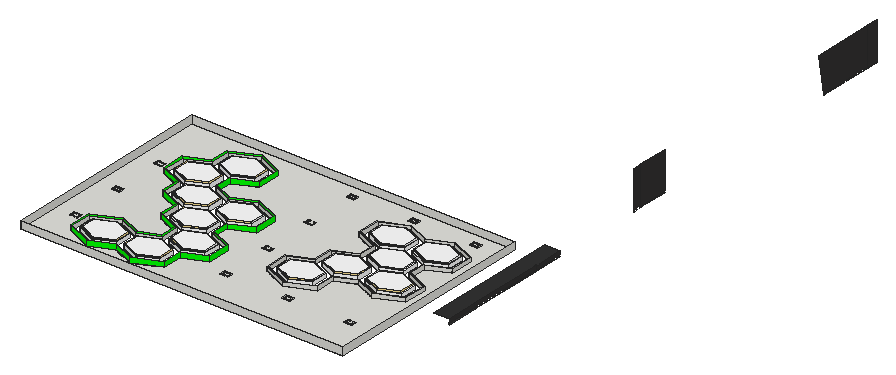
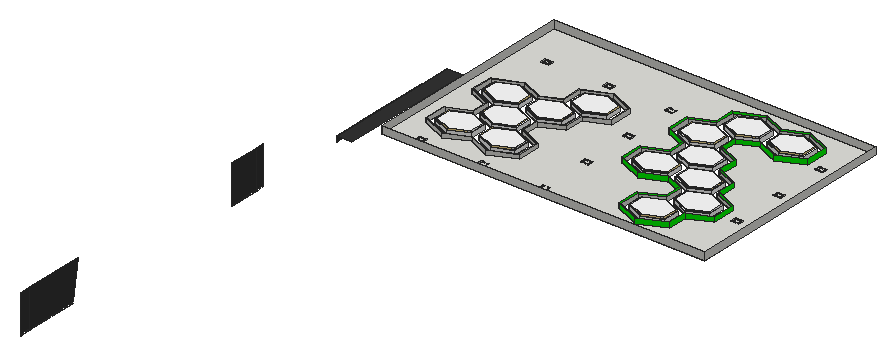
# SketchUp Ruby script. Lengths in inches.
U = 1.inch
M = Sketchup.active_model
def pt(a) = Geom::Point3d.new(a.map { |v| v * U })
def face(e, loops, mat)
  f = e.add_face(loops[0].map { |a| pt(a) })
  loops[1..].each { |l| e.add_face(l.map { |a| pt(a) }).erase! }
  f.material = f.back_material = mat if mat
  f
end
# faces: each face lists its corners as indices into pts; further lists are holes
def faces(e, pts, list, mat = nil) = list.each { |f| face(e, (f[0].is_a?(Array) ? f : [f]).map { |l| l.map { |i| pts[i] } }, mat) }
# xy, xz, yz: faces in a plane at the given z, y or x. An outline is a flat list of corners, or four numbers for a rectangle; further outlines are holes
def ring(l) = l.size == 4 ? [[l[0], l[1]], [l[2], l[1]], [l[2], l[3]], [l[0], l[3]]] : l.each_slice(2).to_a
def flat(e, list, mat, &to3) = list.each { |f| face(e, (f[0].is_a?(Array) ? f : [f]).map { |l| ring(l).map { |u, v| to3.(u, v) } }, mat) }
def xy(e, z, list, mat = nil) = flat(e, list, mat) { |x, y| [x, y, z] }
def xz(e, y, list, mat = nil) = flat(e, list, mat) { |x, z| [x, y, z] }
def yz(e, x, list, mat = nil) = flat(e, list, mat) { |y, z| [x, y, z] }
def lines(e, pts, list) = list.each { |a, b| e.add_line(pt(pts[a]), pt(pts[b])) }
# prism: a flat outline (further loops are holes) pulled along v
def prism(e, loops, v, mat = nil)
  f = face(e, loops, mat); d = Geom::Vector3d.new(v.map { |x| x * U })
  f.pushpull(f.normal.samedirection?(d) ? d.length : -d.length)
end
def box(e, o, s, mat = nil) = prism(e, [[o, [o[0] + s[0], o[1], o[2]], [o[0] + s[0], o[1] + s[1], o[2]], [o[0], o[1] + s[1], o[2]]]], [0, 0, s[2]], mat)
def at(x, y, z, deg = 0) = Geom::Transformation.translation(pt([x, y, z])) * Geom::Transformation.rotation(ORIGIN, Z_AXIS, deg.degrees)
def axes(o, x, y, z) = Geom::Transformation.new([*x, 0, *y, 0, *z, 0, *pt(o).to_a, 1])
def part(name) = M.definitions.add(name)
# library, detail: a bought-in or finely detailed component or shape, given as its bounding box
def library(name, o, s) = part(name).tap { |d| box(d.entities, o, s) }
def detail(e, o, s) = box(e.add_group.entities, o, s)
def put(e, d, t, mat = nil) = e.add_instance(d, t).tap { |i| i.material = mat if mat }
def group(e, t, mat = nil) = e.add_group.tap { |g| g.transformation = t; g.material = mat if mat }.entities
root = M.entities
M.materials.add("False Ceiling Light").color = [250, 224, 145]
M.materials.add("[0128_White]1").color = [255, 255, 255]
M.materials.add("[Color G05]").color = [0, 255, 0]
M.materials.add("[Granite Dark Gray]").color = [51, 50, 50]
c1 = part("Group1089\#2")
p = [[0,0,0],[0,0,-1.54],[-0.31,0,-1.54],[2,-3,0],[-2,-3,0],[2,3,0],
  [2,0,0],[-2,3,0],[0.31,0,-1.54],[-2,0,0],[0,0,-2.5]]
lines(c1.entities,p,[[0,1],[1,2],[3,4],[5,6],[7,5],[1,8],[9,0],[0,6],[8,10],[4,9],[6,3],[2,10],
  [9,7]])
c2 = part("Rectangle Light")
put(c2.entities,c1,at(0,0,0))
c3 = part("Group823\#1")
xy(c3.entities,0,[[-3,-3,3,3]])
put(c3.entities,c2,axes([0,0,-0.01],[1.3627,0,0],[0,1.90637,0],[0,0,1.35135]))
c4 = part("HUY")
xy(c4.entities,0,[[[-1,-1,7,7],[0,0,6,6]]])
xy(c4.entities,0.1,[[0,0,6,6]])
xy(c4.entities,0.6,[[[-1,-1,7,7],[0,0,6,6]]])
xz(c4.entities,-1,[[-1,0,7,0.6]])
xz(c4.entities,0,[[0,0,6,0.1],[0,0.1,6,0.6]])
xz(c4.entities,6,[[0,0,6,0.1],[0,0.1,6,0.6]])
xz(c4.entities,7,[[-1,0,7,0.6]])
yz(c4.entities,-1,[[-1,0,7,0.6]])
yz(c4.entities,0,[[0,0,6,0.1],[0,0.1,6,0.6]])
yz(c4.entities,6,[[0,0,6,0.1],[0,0.1,6,0.6]])
yz(c4.entities,7,[[-1,0,7,0.6]])
put(c4.entities,c3,axes([3,3,0.6],[1,0,0],[0,1,0],[0,0,-1]))
c5 = part("Group849\#3")
xy(c5.entities,0,[[-15.5,-0.5,15.5,0.5]])
c6 = part("Group849\#6")
xy(c6.entities,0,[[-15.5,-0.5,15.5,0.5]])
c7 = part("Group849\#4")
xy(c7.entities,0,[[-15.5,-0.5,15.5,0.5]])
c8 = part("Group849\#5")
xy(c8.entities,0,[[-15.5,-0.5,15.5,0.5]])
c9 = part("HEXAGON")
xy(c9.entities,0,[[15.59,1.15,1,9.58,1,26.42,15.59,34.85,30.18,26.42,30.18,9.58]],"[0128_White]1")
xy(c9.entities,1,[[[15.59,0,0,9,0,27,15.59,36,31.18,27,31.18,9],[15.59,1.15,30.18,9.58,30.18,26.42,15.59,34.85,1,26.42,1,9.58]]],"[0128_White]1")
xy(c9.entities,4,[[15.59,0,31.18,9,31.18,27,15.59,36,0,27,0,9]],"[0128_White]1")
yz(c9.entities,0,[[9,1,27,4]],"[0128_White]1")
yz(c9.entities,1,[[9.58,0,26.42,1]],"[0128_White]1")
yz(c9.entities,30.18,[[9.58,0,26.42,1]],"[0128_White]1")
yz(c9.entities,31.18,[[9,1,27,4]],"[0128_White]1")
p = [[1,9.58,0],[15.59,1.15,0],[15.59,1.15,1],[1,9.58,1],[30.18,9.58,0],[30.18,9.58,1],
  [15.59,34.85,0],[1,26.42,0],[1,26.42,1],[15.59,34.85,1],[30.18,26.42,0],[30.18,26.42,1],
  [0,9,4],[0,9,1],[15.59,0,1],[15.59,0,4],[31.18,9,1],[31.18,9,4],
  [15.59,36,4],[15.59,36,1],[0,27,1],[0,27,4],[31.18,27,4],[31.18,27,1]]
faces(c9.entities,p,[[0,1,2,3],[1,4,5,2],[6,7,8,9],[10,6,9,11]],"False Ceiling Light")
faces(c9.entities,p,[[12,13,14,15],[15,14,16,17],[18,19,20,21],[22,23,19,18]],"[0128_White]1")
put(c9.entities,c5,axes([1,18,0.5],[0,0.5434,0],[0,0,-1],[1,0,0]),"False Ceiling Light")
put(c9.entities,c6,axes([8.29,5.37,0.5],[-0.4706,0.2717,0],[0,0,-1],[0.5,0.86603,0]))
put(c9.entities,c7,axes([22.88,30.63,0.5],[0.4706,-0.2717,0],[0,0,-1],[-0.5,-0.86603,0]))
put(c9.entities,c8,axes([30.18,18,0.5],[0,-0.5434,0],[0,0,-1],[-1,0,0]),"False Ceiling Light")
put(c9.entities,c6,axes([22.88,5.37,0.5],[0.4706,0.2717,0],[0,0,1],[-0.5,0.86603,0]))
put(c9.entities,c6,axes([8.29,30.63,0.5],[-0.4706,-0.2717,0],[0,0,-1],[0.5,-0.86603,0]))
xy(root,248,[[443.875,183,444,207],[443.875,208,444,267],[443.875,268,444,291],[443.875,363,444,369],[443.875,370,444,393],
  [443.875,548.78,444,591],[443.875,592,444,600]],"[Granite Dark Gray]")
xy(root,249,[[443.875,183,444,207],[443.875,208,444,267],[443.875,268,444,291],[443.875,363,444,369],[443.875,370,444,393],
  [443.875,548.61,444,591],[443.875,592,444,600]],"[Granite Dark Gray]")
xy(root,252,[[432,183,444,183,444,207,443.875,207,443.875,208,444,208,444,267,443.875,267,443.875,268,444,268,444,291,432,291]],"[Granite Dark Gray]")
xy(root,253,[[[171,105,423,273],[215.52,114.22,195.74,123.05,195.74,140.72,215.52,149.56,232.56,141.95,246.84,148.33,246.84,161.09,229.81,168.7,229.81,183.91,212.78,191.52,212.78,206.73,195.74,214.24,195.74,232.01,212.78,239.62,212.78,254.83,232.56,263.67,252.34,254.83,252.34,237.16,235.31,229.56,235.31,216.8,249.59,210.42,266.625,218.02,286.41,209.1875,286.41,191.52,269.375,183.91,269.375,171.15,286.41,163.54,286.41,145.875,269.375,138.27,269.375,123.05,249.59,114.22,232.56,121.82],[340.63,149.78,320.85,158.62,320.85,176.39,337.88,183.89,337.88,199.11,354.91,206.72,354.91,219.48,337.88,227.08,337.88,244.75,357.66,253.59,374.7,245.98,391.73,253.59,411.51,244.75,411.51,227.08,394.48,219.48,394.48,206.72,411.51,199.11,411.51,181.4375,391.73,172.6,374.7,180.21,360.41,173.83,360.41,158.62]],[[215.52,114.22,232.56,121.82,249.59,114.22,269.375,123.05,269.375,138.27,286.41,145.875,286.41,163.54,269.375,171.15,269.375,183.91,286.41,191.52,286.41,209.1875,266.625,218.02,249.59,210.42,235.31,216.8,235.31,229.56,252.34,237.16,252.34,254.83,232.56,263.67,212.78,254.83,212.78,239.62,195.74,232.01,195.74,214.24,212.78,206.73,212.78,191.52,229.81,183.91,229.81,168.7,246.84,161.09,246.84,148.33,232.56,141.95,215.52,149.56,195.74,140.72,195.74,123.05],[215.52,115.03,196.66,123.46,196.66,140.3125,215.52,148.74,232.56,141.13,247.76,147.92,247.76,161.5,230.73,169.1,230.73,184.32,213.69,191.93,213.69,207.15,196.66,214.65,196.66,231.6,213.69,239.21,213.69,254.42,232.56,262.85,251.42,254.42,251.42,237.57,234.39,229.97,234.39,216.39,249.59,209.6,266.625,217.21,285.49,208.78,285.49,191.93,268.46,184.32,268.46,170.74,285.49,163.13,285.49,146.28,268.46,138.67,268.46,123.46,249.59,115.03,232.56,122.64]],[[340.63,149.78,360.41,158.62,360.41,173.83,374.7,180.21,391.73,172.6,411.51,181.4375,411.51,199.11,394.48,206.72,394.48,219.48,411.51,227.08,411.51,244.75,391.73,253.59,374.7,245.98,357.66,253.59,337.88,244.75,337.88,227.08,354.91,219.48,354.91,206.72,337.88,199.11,337.88,183.89,320.85,176.39,320.85,158.62],[340.63,150.6,321.76,159.02,321.76,175.98,338.8,183.48,338.8,198.7,355.83,206.31,355.83,219.88,338.8,227.49,338.8,244.34,357.66,252.77,374.7,245.16,391.73,252.77,410.6,244.34,410.6,227.49,393.5625,219.88,393.5625,206.31,410.6,198.7,410.6,181.85,391.73,173.42,374.7,181.03,359.5,174.24,359.5,159.02]]])
xz(root,105,[[171,253,423,259]])
xz(root,207,[[443.875,249,444,252]],"[Granite Dark Gray]")
xz(root,208,[[443.875,249,444,252]],"[Granite Dark Gray]")
xz(root,267,[[443.875,249,444,252]],"[Granite Dark Gray]")
xz(root,268,[[443.875,249,444,252]],"[Granite Dark Gray]")
xz(root,273,[[171,253,423,259]])
xz(root,369,[[443.875,249,444,278]],"[Granite Dark Gray]")
xz(root,370,[[443.875,249,444,278]],"[Granite Dark Gray]")
xz(root,591,[[443.875,249,444,278]],"[Granite Dark Gray]")
xz(root,592,[[443.875,249,444,278]],"[Granite Dark Gray]")
yz(root,171,[[105,253,273,259]])
yz(root,195.74,[[123.05,253,140.72,257],[214.24,253,232.01,257]],"[Color G05]")
yz(root,196.66,[[123.46,253,140.3125,256],[214.65,253,231.6,256]])
yz(root,212.78,[[191.52,253,206.73,257],[239.62,253,254.83,257]],"[Color G05]")
yz(root,213.69,[[191.93,253,207.15,256],[239.21,253,254.42,256]])
yz(root,229.81,[[168.7,253,183.91,257]],"[Color G05]")
yz(root,230.73,[[169.1,253,184.32,256]])
yz(root,234.39,[[216.39,253,229.97,256]])
yz(root,235.31,[[216.8,253,229.56,257]],"[Color G05]")
yz(root,246.84,[[148.33,253,161.09,257]],"[Color G05]")
yz(root,247.76,[[147.92,253,161.5,256]])
yz(root,251.42,[[237.57,253,254.42,256]])
yz(root,252.34,[[237.16,253,254.83,257]],"[Color G05]")
yz(root,268.46,[[123.46,253,138.67,256],[170.74,253,184.32,256]])
yz(root,269.375,[[123.05,253,138.27,257],[171.15,253,183.91,257]],"[Color G05]")
yz(root,285.49,[[146.28,253,163.13,256],[191.93,253,208.78,256]])
yz(root,286.41,[[145.875,253,163.54,257],[191.52,253,209.1875,257]],"[Color G05]")
yz(root,320.85,[[158.62,253,176.39,256]])
yz(root,321.76,[[159.02,253,175.98,256]])
yz(root,337.88,[[183.89,253,199.11,256],[227.08,253,244.75,256]])
yz(root,338.8,[[183.48,253,198.7,256],[227.49,253,244.34,256]])
yz(root,354.91,[[206.72,253,219.48,256]])
yz(root,355.83,[[206.31,253,219.88,256]])
yz(root,359.5,[[159.02,253,174.24,256]])
yz(root,360.41,[[158.62,253,173.83,256]])
yz(root,393.5625,[[206.31,253,219.88,256]])
yz(root,394.48,[[206.72,253,219.48,256]])
yz(root,410.6,[[181.85,253,198.7,256],[227.49,253,244.34,256]])
yz(root,411.51,[[181.4375,253,199.11,256],[227.08,253,244.75,256]])
yz(root,423,[[105,253,273,259]])
yz(root,444,[[183,249,207,252],[208,249,267,252],[268,249,291,252],[363,249,369,278],[370,249,393,278],
  [548.61,249,591,249,591,278,543.57,278],[592,249,600,278]],"[Granite Dark Gray]")
p = [[215.52,114.22,257],[195.74,123.05,257],[195.74,123.05,253],[215.52,114.22,253],[232.56,121.82,257],[232.56,121.82,253],
  [249.59,114.22,257],[249.59,114.22,253],[269.375,123.05,257],[269.375,123.05,253],[215.52,115.03,256],[196.66,123.46,256],
  [196.66,123.46,253],[215.52,115.03,253],[232.56,122.64,256],[232.56,122.64,253],[249.59,115.03,256],[249.59,115.03,253],
  [268.46,123.46,256],[268.46,123.46,253],[286.41,145.875,257],[269.375,138.27,257],[269.375,138.27,253],[286.41,145.875,253],
  [285.49,146.28,256],[268.46,138.67,256],[268.46,138.67,253],[285.49,146.28,253],[196.66,140.3125,256],[215.52,148.74,256],
  [215.52,148.74,253],[196.66,140.3125,253],[215.52,149.56,257],[215.52,149.56,253],[195.74,140.72,253],[195.74,140.72,257],
  [232.56,141.13,256],[232.56,141.13,253],[247.76,147.92,256],[247.76,147.92,253],[232.56,141.95,257],[232.56,141.95,253],
  [246.84,148.33,257],[246.84,148.33,253],[340.63,149.78,253],[340.63,149.78,256],[320.85,158.62,256],[320.85,158.62,253],
  [360.41,158.62,253],[360.41,158.62,256],[340.63,150.6,256],[321.76,159.02,256],[321.76,159.02,253],[340.63,150.6,253],
  [359.5,159.02,256],[359.5,159.02,253],[229.81,168.7,257],[229.81,168.7,253],[246.84,161.09,253],[246.84,161.09,257],
  [247.76,161.5,256],[230.73,169.1,256],[230.73,169.1,253],[247.76,161.5,253],[268.46,170.74,256],[285.49,163.13,256],
  [285.49,163.13,253],[268.46,170.74,253],[269.375,171.15,257],[286.41,163.54,257],[286.41,163.54,253],[269.375,171.15,253],
  [391.73,172.6,253],[391.73,172.6,256],[374.7,180.21,256],[374.7,180.21,253],[411.51,181.4375,253],[411.51,181.4375,256],
  [391.73,173.42,256],[374.7,181.03,256],[374.7,181.03,253],[391.73,173.42,253],[410.6,181.85,256],[410.6,181.85,253],
  [360.41,173.83,256],[360.41,173.83,253],[359.5,174.24,256],[359.5,174.24,253],[321.76,175.98,256],[338.8,183.48,256],
  [338.8,183.48,253],[321.76,175.98,253],[320.85,176.39,253],[320.85,176.39,256],[337.88,183.89,256],[337.88,183.89,253],
  [212.78,191.52,257],[212.78,191.52,253],[229.81,183.91,253],[229.81,183.91,257],[286.41,191.52,257],[269.375,183.91,257],
  [269.375,183.91,253],[286.41,191.52,253],[230.73,184.32,256],[213.69,191.93,256],[213.69,191.93,253],[230.73,184.32,253],
  [285.49,191.93,256],[268.46,184.32,256],[268.46,184.32,253],[285.49,191.93,253],[338.8,198.7,256],[355.83,206.31,256],
  [355.83,206.31,253],[338.8,198.7,253],[393.5625,206.31,256],[410.6,198.7,256],[410.6,198.7,253],[393.5625,206.31,253],
  [337.88,199.11,253],[337.88,199.11,256],[354.91,206.72,256],[354.91,206.72,253],[394.48,206.72,253],[394.48,206.72,256],
  [411.51,199.11,256],[411.51,199.11,253],[195.74,214.24,257],[195.74,214.24,253],[212.78,206.73,253],[212.78,206.73,257],
  [213.69,207.15,256],[196.66,214.65,256],[196.66,214.65,253],[213.69,207.15,253],[266.625,217.21,256],[285.49,208.78,256],
  [285.49,208.78,253],[266.625,217.21,253],[266.625,218.02,257],[286.41,209.1875,257],[286.41,209.1875,253],[266.625,218.02,253],
  [234.39,216.39,256],[249.59,209.6,256],[249.59,209.6,253],[234.39,216.39,253],[235.31,216.8,257],[249.59,210.42,257],
  [249.59,210.42,253],[235.31,216.8,253],[354.91,219.48,253],[354.91,219.48,256],[337.88,227.08,256],[337.88,227.08,253],
  [411.51,227.08,253],[411.51,227.08,256],[394.48,219.48,256],[394.48,219.48,253],[355.83,219.88,256],[338.8,227.49,256],
  [338.8,227.49,253],[355.83,219.88,253],[410.6,227.49,256],[393.5625,219.88,256],[393.5625,219.88,253],[410.6,227.49,253],
  [252.34,237.16,257],[235.31,229.56,257],[235.31,229.56,253],[252.34,237.16,253],[251.42,237.57,256],[234.39,229.97,256],
  [234.39,229.97,253],[251.42,237.57,253],[196.66,231.6,256],[213.69,239.21,256],[213.69,239.21,253],[196.66,231.6,253],
  [212.78,239.62,257],[212.78,239.62,253],[195.74,232.01,253],[195.74,232.01,257],[338.8,244.34,256],[357.66,252.77,256],
  [357.66,252.77,253],[338.8,244.34,253],[391.73,252.77,256],[410.6,244.34,256],[410.6,244.34,253],[391.73,252.77,253],
  [337.88,244.75,253],[337.88,244.75,256],[357.66,253.59,256],[357.66,253.59,253],[391.73,253.59,253],[391.73,253.59,256],
  [411.51,244.75,256],[411.51,244.75,253],[374.7,245.16,256],[374.7,245.16,253],[374.7,245.98,256],[374.7,245.98,253],
  [213.69,254.42,256],[232.56,262.85,256],[232.56,262.85,253],[213.69,254.42,253],[251.42,254.42,256],[251.42,254.42,253],
  [212.78,254.83,257],[232.56,263.67,257],[232.56,263.67,253],[212.78,254.83,253],[252.34,254.83,257],[252.34,254.83,253]]
faces(root,p,[[0,1,2,3],[4,0,3,5],[6,4,5,7],[8,6,7,9],[20,21,22,23],[32,33,34,35],[40,41,33,32],[42,43,41,40],
  [56,57,58,59],[68,69,70,71],[96,97,98,99],[100,101,102,103],[128,129,130,131],[140,141,142,143],[148,149,150,151],[149,140,143,150],
  [168,169,170,171],[180,181,182,183],[210,211,212,213],[211,214,215,212]],"[Color G05]")
faces(root,p,[[10,11,12,13],[14,10,13,15],[16,14,15,17],[18,16,17,19],[24,25,26,27],[28,29,30,31],[29,36,37,30],[36,38,39,37],
  [44,45,46,47],[48,49,45,44],[50,51,52,53],[54,50,53,55],[60,61,62,63],[64,65,66,67],[72,73,74,75],[76,77,73,72],
  [78,79,80,81],[82,78,81,83],[75,74,84,85],[79,86,87,80],[88,89,90,91],[92,93,94,95],[104,105,106,107],[108,109,110,111],
  [112,113,114,115],[116,117,118,119],[120,121,122,123],[124,125,126,127],[132,133,134,135],[136,137,138,139],[144,145,146,147],[145,136,139,146],
  [152,153,154,155],[156,157,158,159],[160,161,162,163],[164,165,166,167],[172,173,174,175],[176,177,178,179],[184,185,186,187],[188,189,190,191],
  [192,193,194,195],[196,197,198,199],[185,200,201,186],[200,188,191,201],[195,194,202,203],[203,202,197,196],[204,205,206,207],[205,208,209,206]])
put(root,c4,axes([398.11,138.59,253],[0.73384,0,0],[0,0.52456,0],[0,0,-0.74]))
put(root,c4,axes([301.67,261.61,253],[0.73384,0,0],[0,0.52456,0],[0,0,-0.74]))
put(root,c4,axes([183.92,179.54,253],[0.73384,0,0],[0,0.52456,0],[0,0,-0.74]))
put(root,c4,axes([183.92,138.59,253],[0.73384,0,0],[0,0.52456,0],[0,0,-0.74]))
put(root,c4,axes([301.67,138.4375,253],[0.73384,0,0],[0,0.52456,0],[0,0,-0.74]))
put(root,c4,axes([349.89,261.61,253],[0.73384,0,0],[0,0.52456,0],[0,0,-0.74]))
put(root,c4,axes([301.67,179.39,253],[0.73384,0,0],[0,0.52456,0],[0,0,-0.74]))
put(root,c4,axes([398.11,261.61,253],[0.73384,0,0],[0,0.52456,0],[0,0,-0.74]))
put(root,c4,axes([301.67,220.5,253],[0.73384,0,0],[0,0.52456,0],[0,0,-0.74]))
put(root,c4,axes([349.89,138.4375,253],[0.73384,0,0],[0,0.52456,0],[0,0,-0.74]))
put(root,c4,axes([183.92,220.65,253],[0.73384,0,0],[0,0.52456,0],[0,0,-0.74]))
put(root,c9,axes([218.27,233.24,257],[0.91636,0,0],[0,0.70886,0],[0,0,-1]))
put(root,c9,axes([252.34,187.59,257],[0.91636,0,0],[0,0.70886,0],[0,0,-1]))
put(root,c9,axes([201.24,210.42,257],[0.91636,0,0],[0,0.70886,0],[0,0,-1]))
put(root,c9,axes([326.34,154.69,257],[0.91636,0,0],[0,0.70886,0],[0,0,-1]))
put(root,c9,axes([343.38,223.16,257],[0.91636,0,0],[0,0.70886,0],[0,0,-1]))
put(root,c9,axes([377.45,223.16,257],[0.91636,0,0],[0,0.70886,0],[0,0,-1]))
put(root,c9,axes([377.45,177.51,257],[0.91636,0,0],[0,0.70886,0],[0,0,-1]))
put(root,c9,axes([235.31,119.125,257],[0.91636,0,0],[0,0.70886,0],[0,0,-1]))
put(root,c9,axes([201.24,119.125,257],[0.91636,0,0],[0,0.70886,0],[0,0,-1]))
put(root,c9,axes([252.34,141.95,257],[0.91636,0,0],[0,0.70886,0],[0,0,-1]))
put(root,c9,axes([343.38,177.51,257],[0.91636,0,0],[0,0.70886,0],[0,0,-1]))
put(root,c9,axes([218.27,187.59,257],[0.91636,0,0],[0,0.70886,0],[0,0,-1]))
put(root,c9,axes([235.31,164.77,257],[0.91636,0,0],[0,0.70886,0],[0,0,-1]))
put(root,c9,axes([360.41,200.34,257],[0.91636,0,0],[0,0.70886,0],[0,0,-1]))
